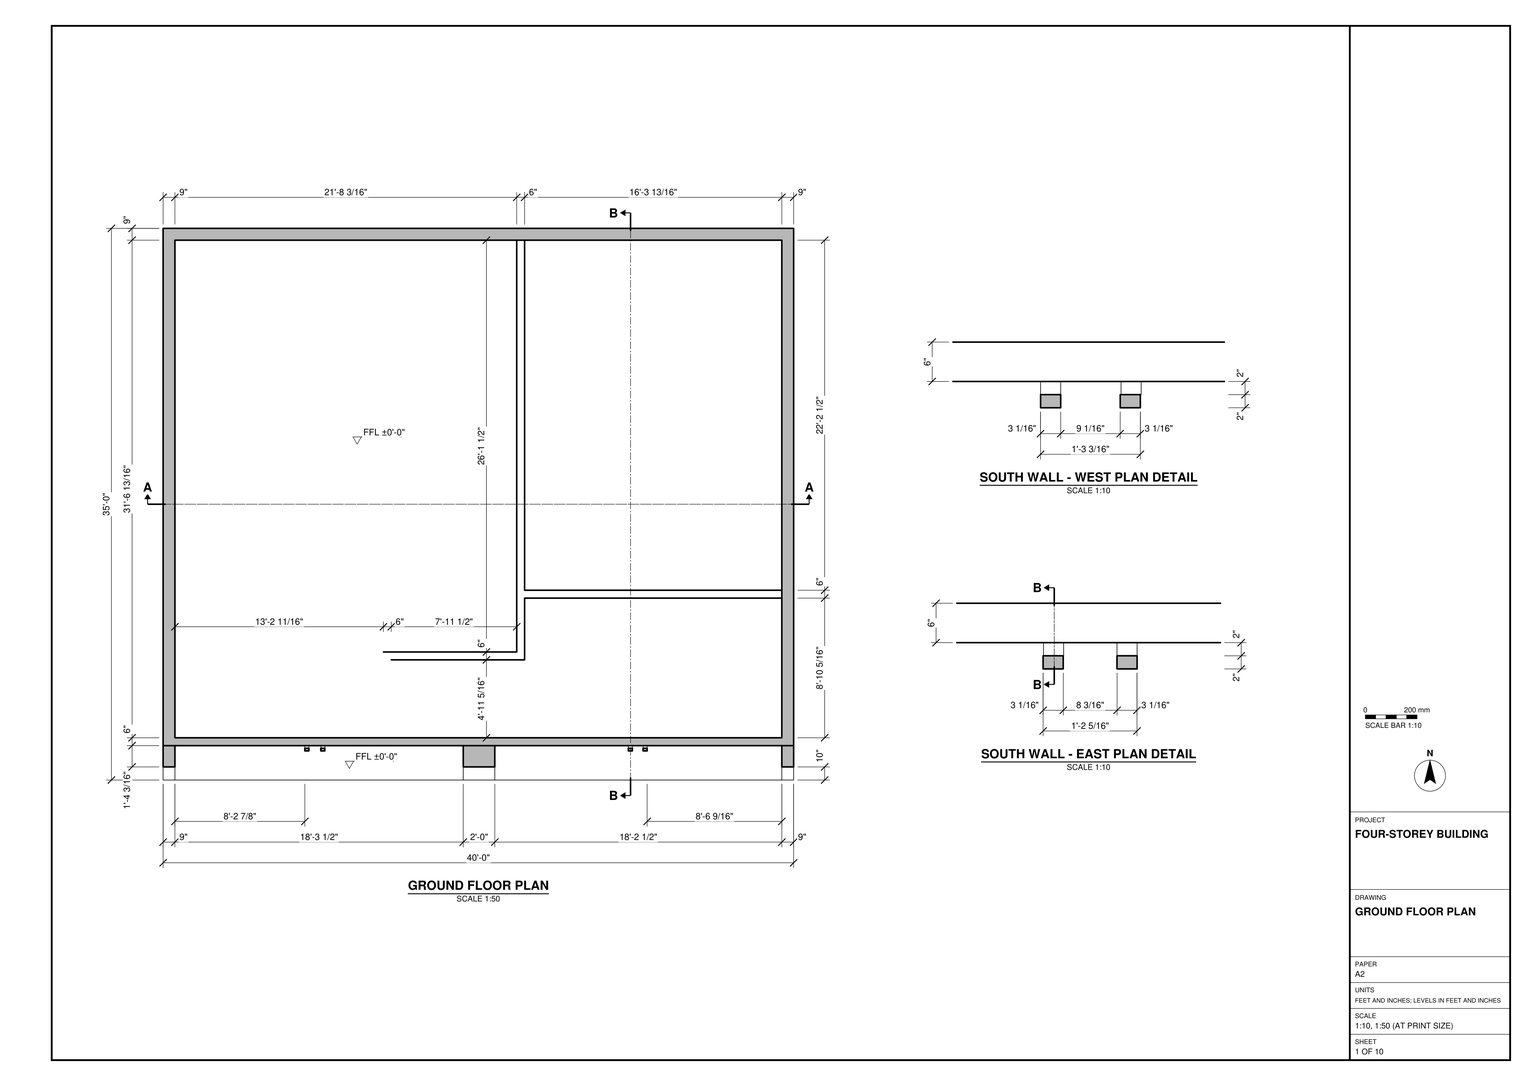
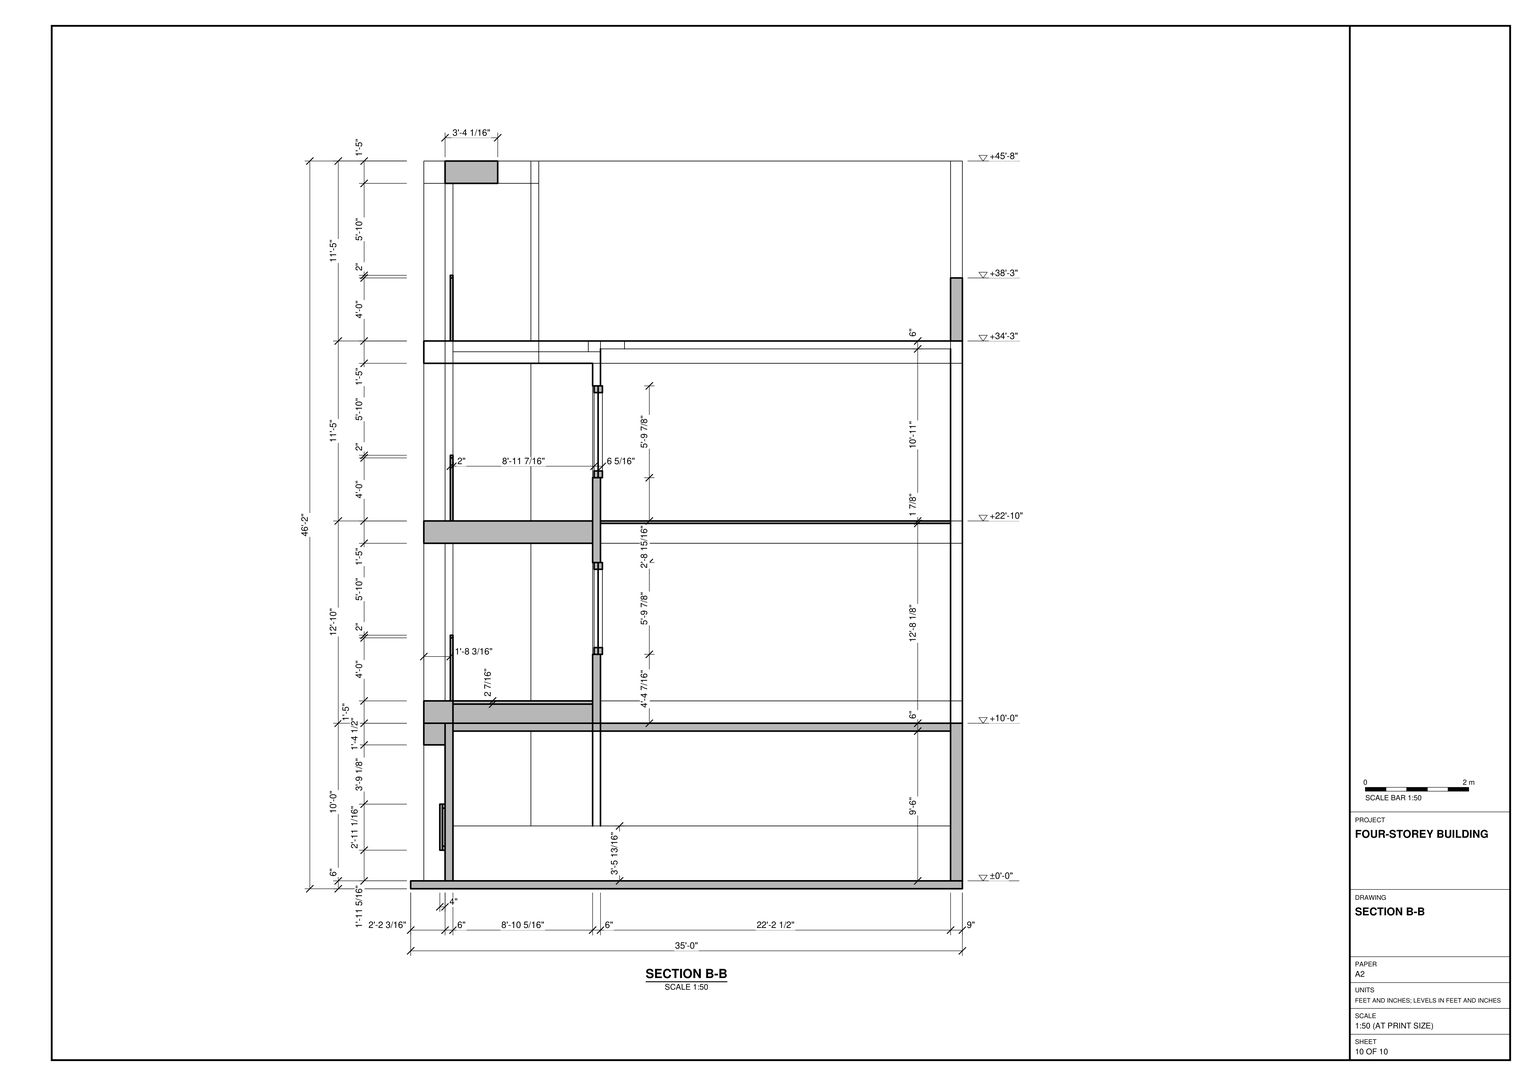
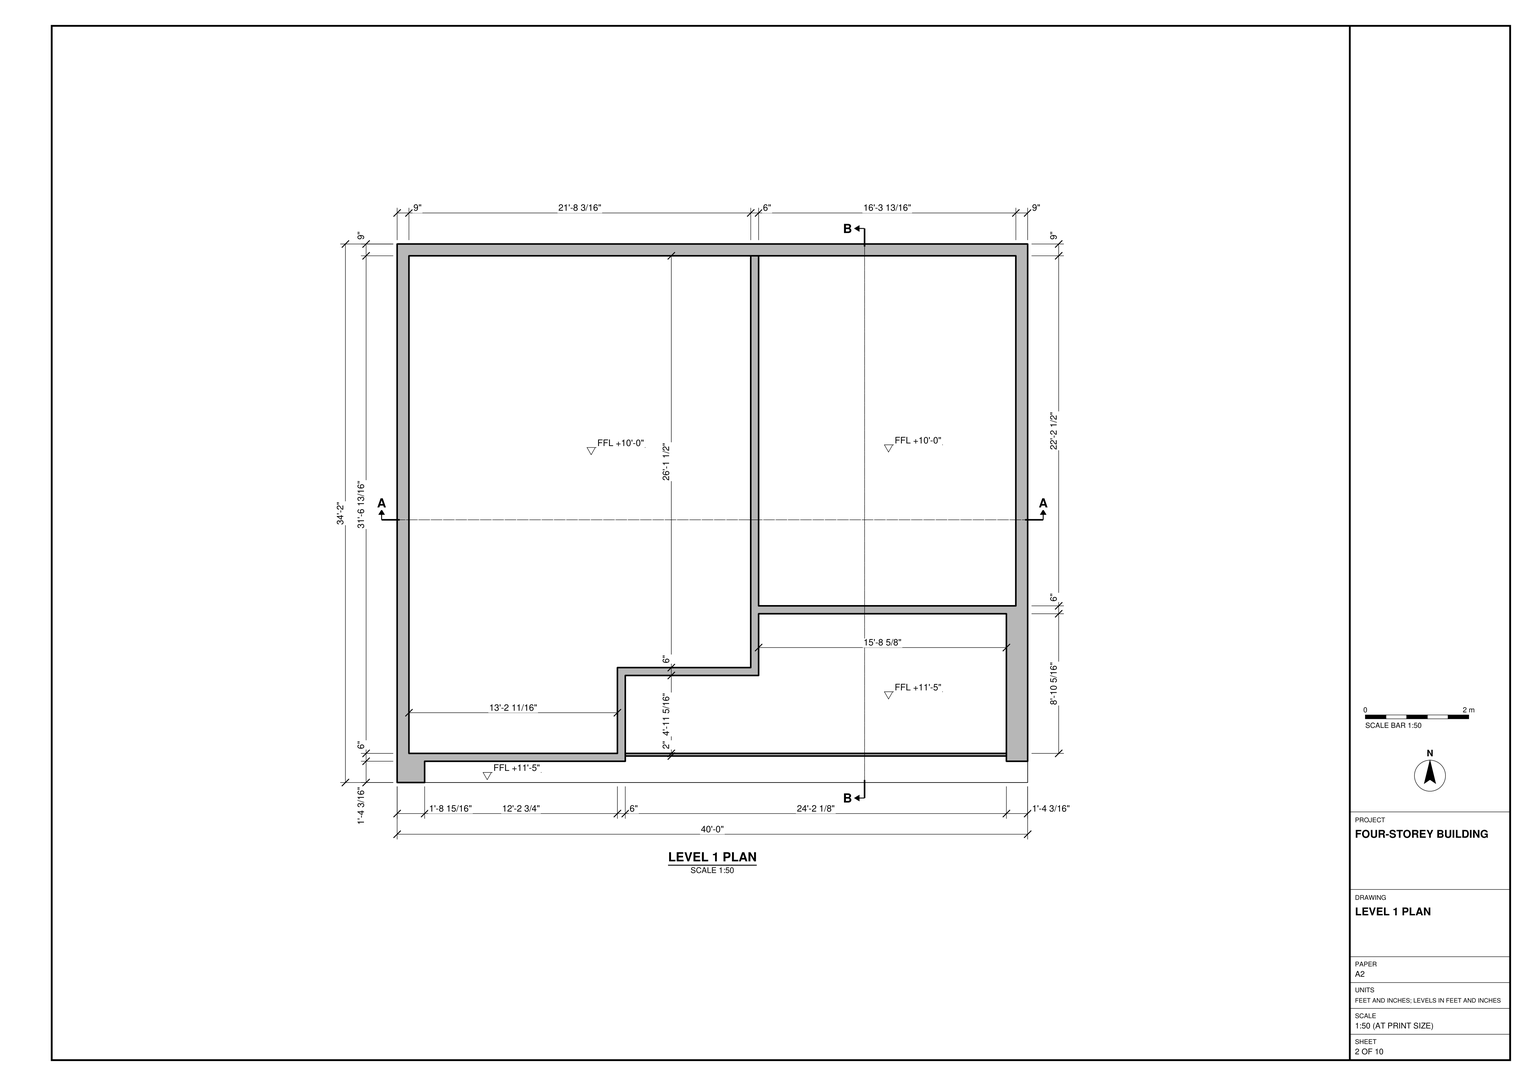
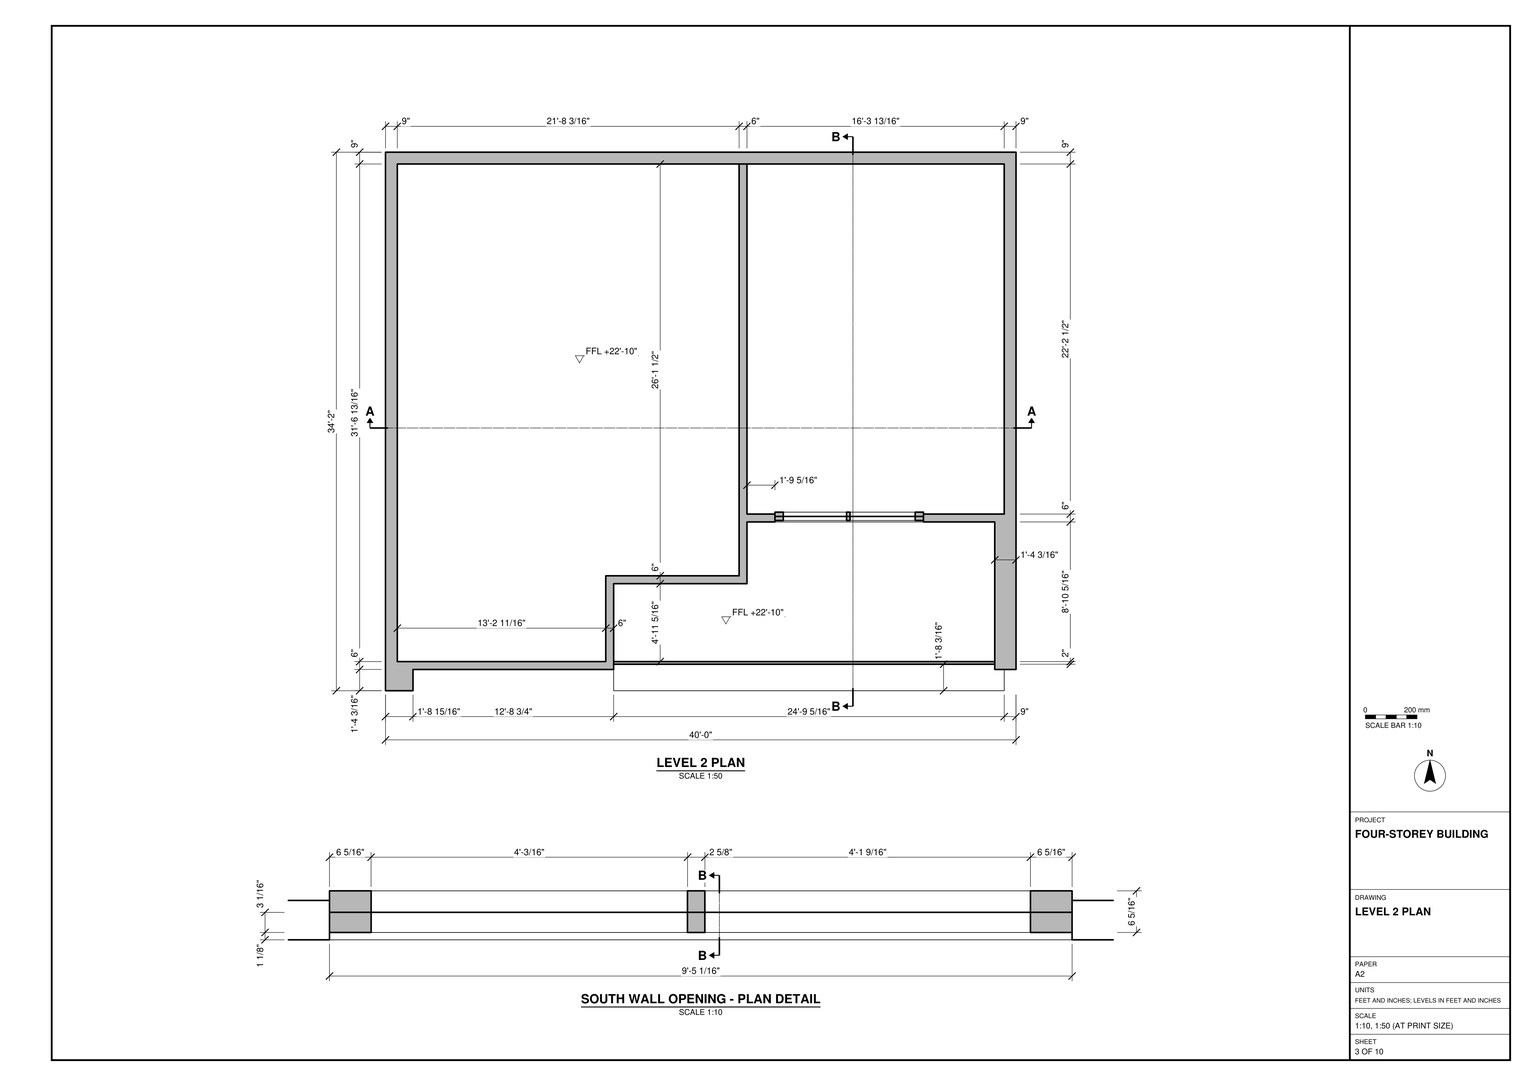
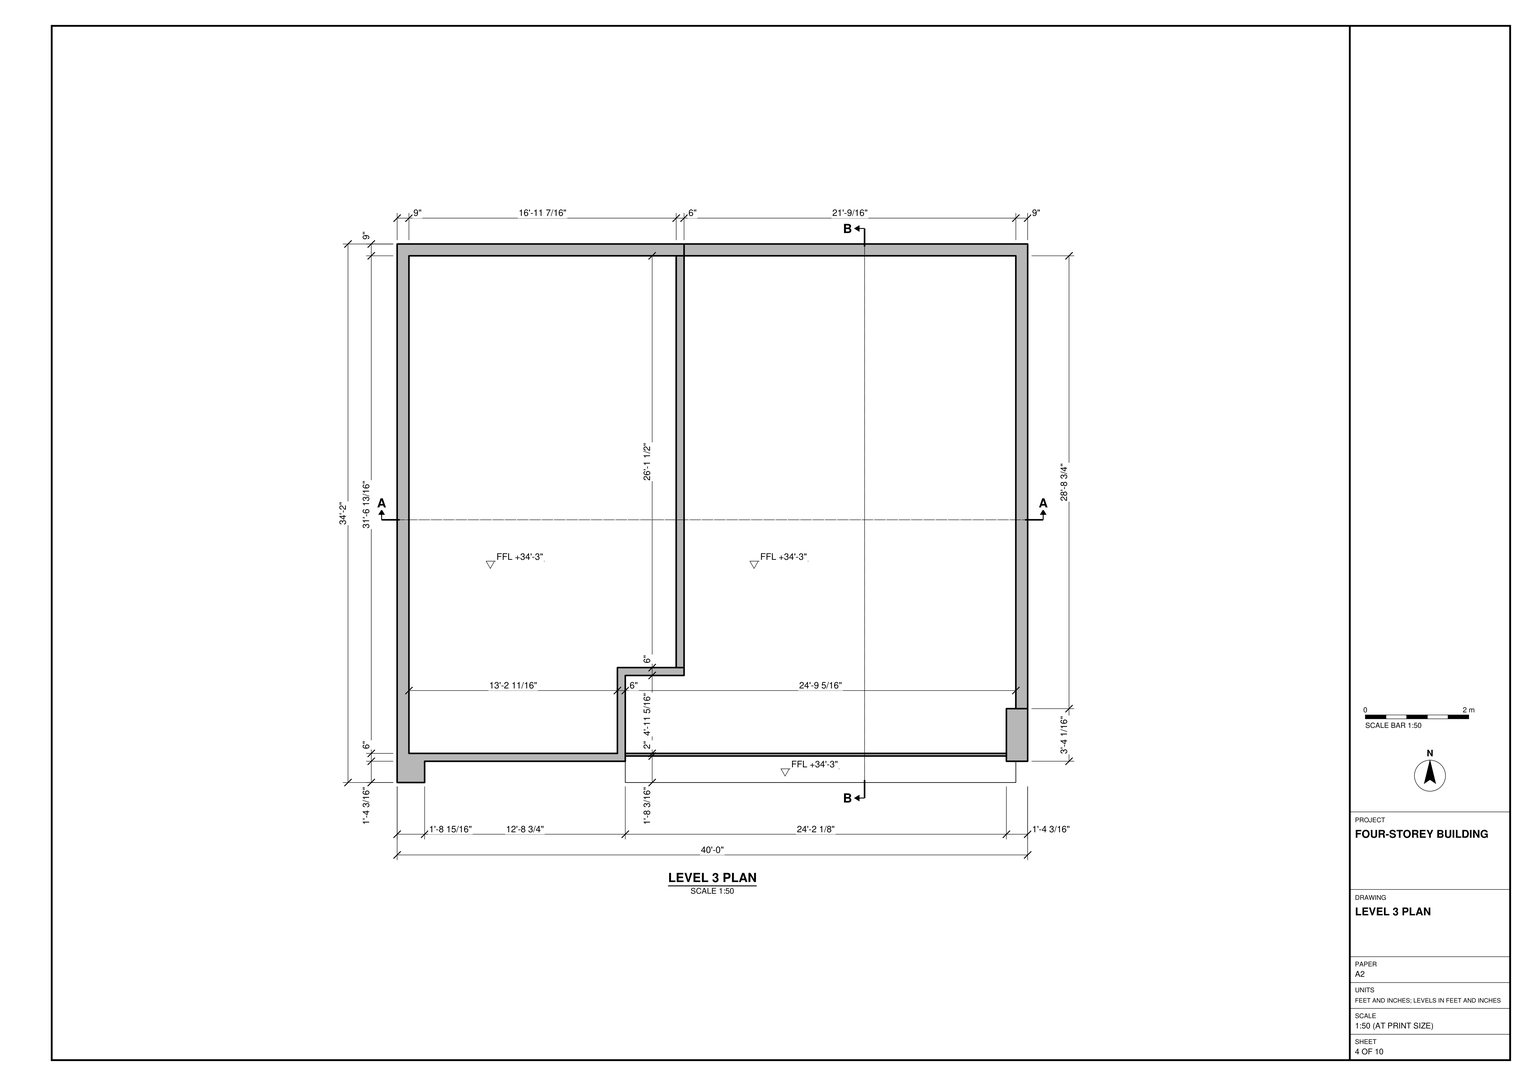
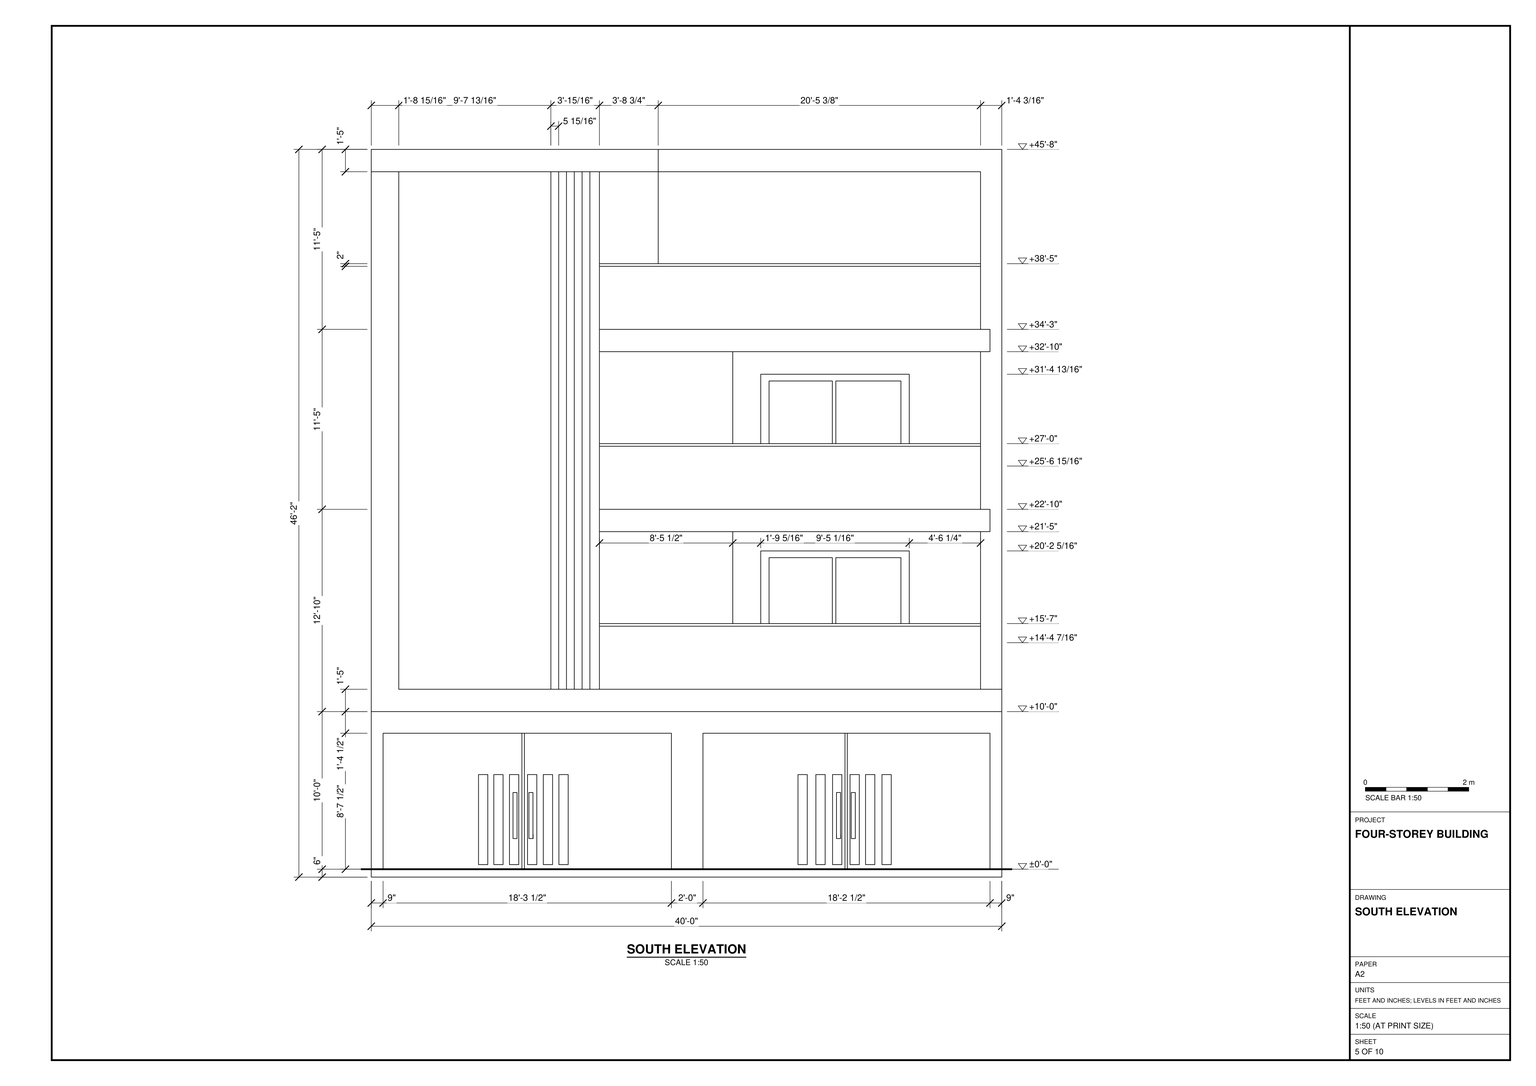
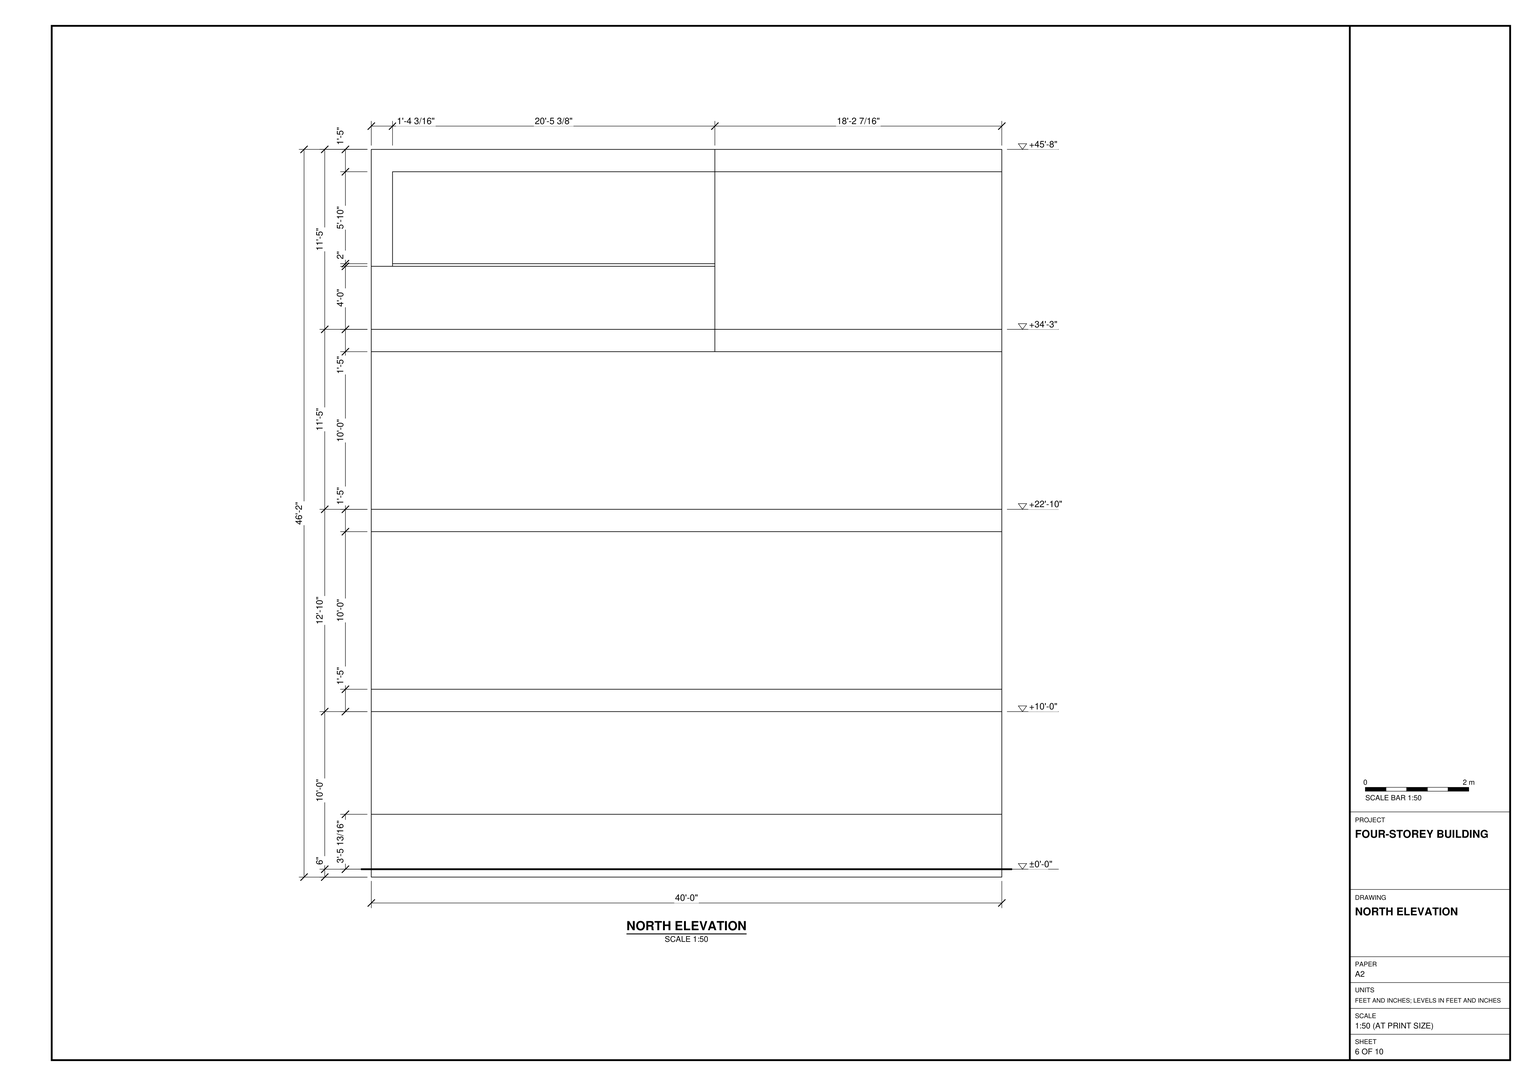
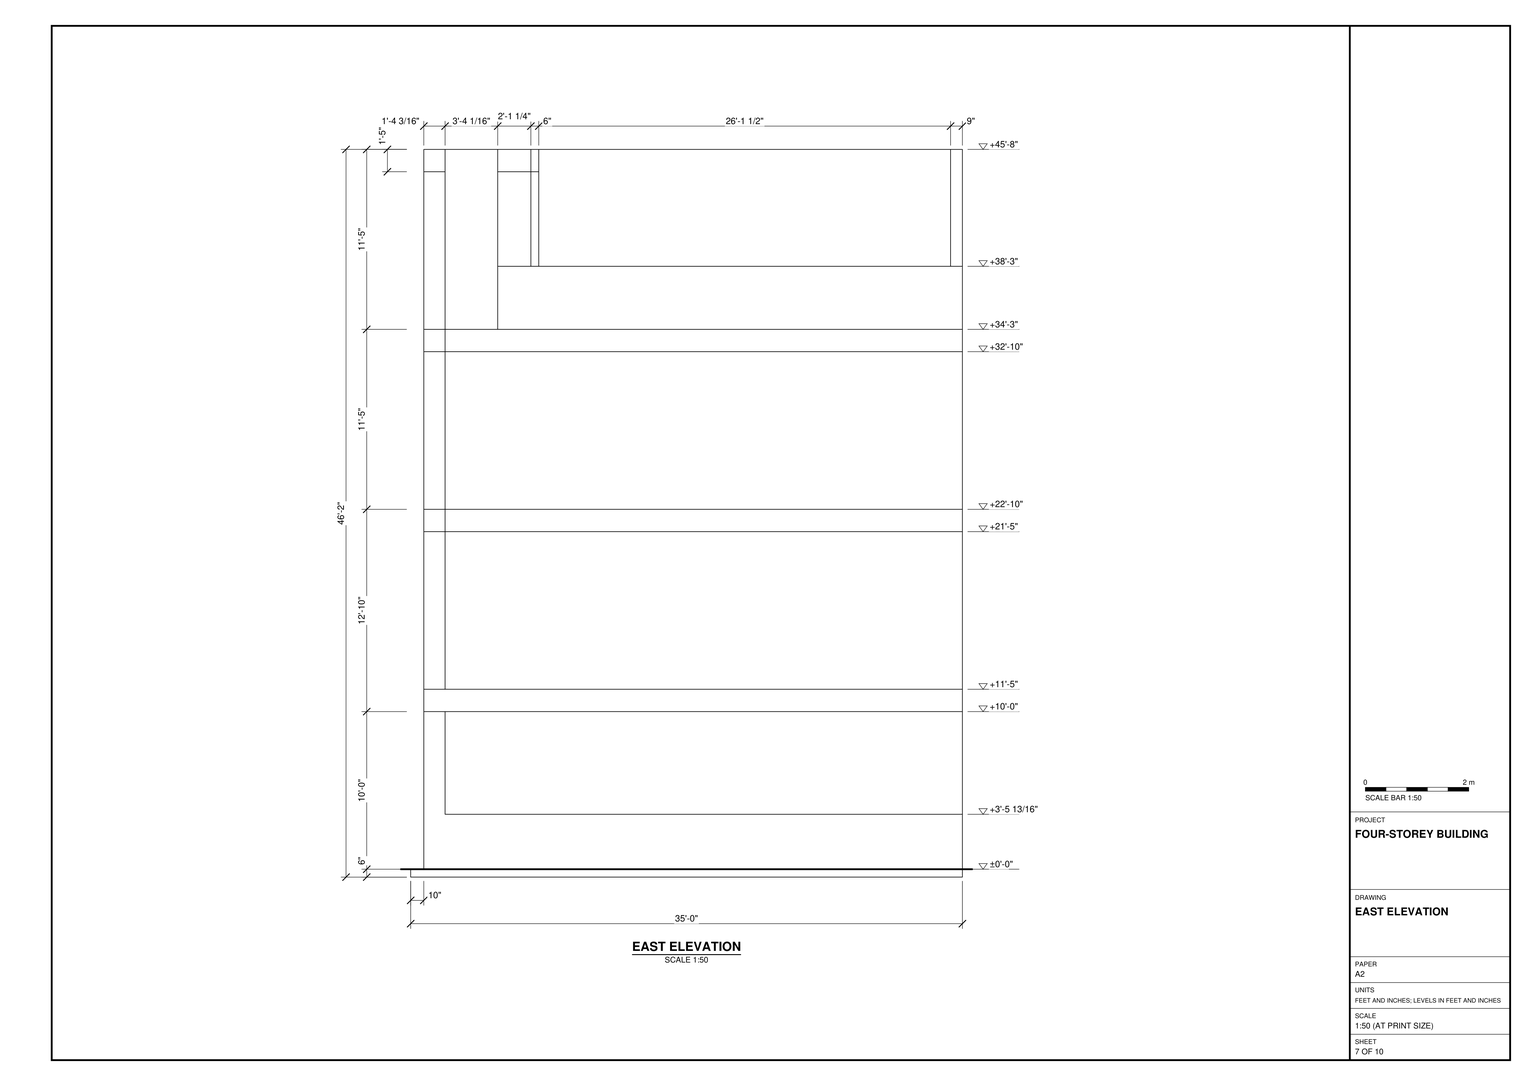
Build the four-storey building in SketchUp from task_files/diagram_01.pdf. Work in feet and inches. Set the east–west width along X to 40'-0" and the north–south depth along Y to 35'-0". The overall height is 46'-2", measured from the underside of the ground slab, not from its finished floor. Set the finished floor levels to ±0'-0", +10'-0", +22'-10" and +34'-3".

Use each floor plan for its own wall and slab outlines. Follow the wall thicknesses as drawn, including the 9" north and side walls and the 6" partitions where indicated. At the south frontage, distinguish the projecting ground slab from the stepped wall line above. Model the raised front floor area on level 1 at +11'-5" rather than continuing the +10'-0" floor through it. Use the sections to resolve slab depths, openings, guards and the roofline. Model stairs, built-in joinery and main furniture only where shown.

Keep walls, slabs and roof elements in separate groups or components. Group each furniture or joinery piece separately and use components for repeated parts. Decor and loose items, if shown, may be any suitable library components. Save one SketchUp model as output_files/four_storey_building_with_its_stepped_south_frontage.skp.

# SketchUp Ruby script. Lengths in inches.
U = 1.inch
M = Sketchup.active_model
def pt(a) = Geom::Point3d.new(a.map { |v| v * U })
def face(e, loops, mat)
  f = e.add_face(loops[0].map { |a| pt(a) })
  loops[1..].each { |l| e.add_face(l.map { |a| pt(a) }).erase! }
  f.material = f.back_material = mat if mat
  f
end
# faces: each face lists its corners as indices into pts; further lists are holes
def faces(e, pts, list, mat = nil) = list.each { |f| face(e, (f[0].is_a?(Array) ? f : [f]).map { |l| l.map { |i| pts[i] } }, mat) }
# xy, xz, yz: faces in a plane at the given z, y or x. An outline is a flat list of corners, or four numbers for a rectangle; further outlines are holes
def ring(l) = l.size == 4 ? [[l[0], l[1]], [l[2], l[1]], [l[2], l[3]], [l[0], l[3]]] : l.each_slice(2).to_a
def flat(e, list, mat, &to3) = list.each { |f| face(e, (f[0].is_a?(Array) ? f : [f]).map { |l| ring(l).map { |u, v| to3.(u, v) } }, mat) }
def xy(e, z, list, mat = nil) = flat(e, list, mat) { |x, y| [x, y, z] }
def xz(e, y, list, mat = nil) = flat(e, list, mat) { |x, z| [x, y, z] }
def yz(e, x, list, mat = nil) = flat(e, list, mat) { |y, z| [x, y, z] }
def lines(e, pts, list) = list.each { |a, b| e.add_line(pt(pts[a]), pt(pts[b])) }
# prism: a flat outline (further loops are holes) pulled along v
def prism(e, loops, v, mat = nil)
  f = face(e, loops, mat); d = Geom::Vector3d.new(v.map { |x| x * U })
  f.pushpull(f.normal.samedirection?(d) ? d.length : -d.length)
end
def box(e, o, s, mat = nil) = prism(e, [[o, [o[0] + s[0], o[1], o[2]], [o[0] + s[0], o[1] + s[1], o[2]], [o[0], o[1] + s[1], o[2]]]], [0, 0, s[2]], mat)
def at(x, y, z, deg = 0) = Geom::Transformation.translation(pt([x, y, z])) * Geom::Transformation.rotation(ORIGIN, Z_AXIS, deg.degrees)
def axes(o, x, y, z) = Geom::Transformation.new([*x, 0, *y, 0, *z, 0, *pt(o).to_a, 1])
def part(name) = M.definitions.add(name)
# library, detail: a bought-in or finely detailed component or shape, given as its bounding box
def library(name, o, s) = part(name).tap { |d| box(d.entities, o, s) }
def detail(e, o, s) = box(e.add_group.entities, o, s)
def put(e, d, t, mat = nil) = e.add_instance(d, t).tap { |i| i.material = mat if mat }
def group(e, t, mat = nil) = e.add_group.tap { |g| g.transformation = t; g.material = mat if mat }.entities
root = M.entities
M.materials.add("[Color B08]").color = [74, 25, 0]
M.materials.add("[Granite Brown]").color = [126, 104, 91]
M.materials.add("[Metal Corrugated Shiny]").color = [193, 193, 70]
M.materials.add("[Metal Silver]").color = [234, 233, 238]
M.materials.add("[Stone Brushed Khaki]").color = [226, 197, 133]
M.materials.add("[Translucent Glass Gray]").color = [128, 128, 128]
M.materials["[Translucent Glass Gray]"].alpha = 0.5
M.materials.add("[Wood Cherry Original]").color = [152, 86, 42]
M.materials.add("[Wood Floor]").color = [155, 105, 61]
M.materials.add("[Wood Veneer 01]").color = [120, 70, 37]
c1 = part("Group\#1")
xy(c1.entities,0,[[0,0,184.75,6.5625],[0,6.5625,184.75,13.5625]],"[Color B08]")
xy(c1.entities,10.36,[[10.36,0,89.06,6.5625],[93.39,0,174.39,6.5625],[10.36,6.5625,89.06,13.5625],[93.39,6.5625,174.39,13.5625]],"[Color B08]")
xy(c1.entities,131.02,[[10.36,0,89.06,6.5625],[93.39,0,174.39,6.5625],[10.36,6.5625,89.06,13.5625],[93.39,6.5625,174.39,13.5625]],"[Color B08]")
xy(c1.entities,141.375,[[0,0,184.75,6.5625],[0,6.5625,184.75,13.5625]],"[Color B08]")
xz(c1.entities,0,[[[0,0,184.75,141.375],[93.39,10.36,174.39,131.02],[10.36,10.36,89.06,131.02]]],"[Color B08]")
xz(c1.entities,6.5625,[[[0,0,184.75,141.375],[93.39,10.36,174.39,131.02],[10.36,10.36,89.06,131.02]]],"[Color B08]")
xz(c1.entities,6.5625,[[10.36,10.36,89.06,131.02],[93.39,10.36,174.39,131.02]],"[Translucent Glass Gray]")
xz(c1.entities,13.5625,[[[0,0,184.75,141.375],[93.39,10.36,174.39,131.02],[10.36,10.36,89.06,131.02]]],"[Color B08]")
yz(c1.entities,0,[[0,0,6.5625,141.375],[6.5625,0,13.5625,141.375]],"[Color B08]")
yz(c1.entities,10.36,[[0,10.36,6.5625,131.02],[6.5625,10.36,13.5625,131.02]],"[Color B08]")
yz(c1.entities,89.06,[[0,10.36,6.5625,131.02],[6.5625,10.36,13.5625,131.02]],"[Color B08]")
yz(c1.entities,93.39,[[0,10.36,6.5625,131.02],[6.5625,10.36,13.5625,131.02]],"[Color B08]")
yz(c1.entities,174.39,[[0,10.36,6.5625,131.02],[6.5625,10.36,13.5625,131.02]],"[Color B08]")
yz(c1.entities,184.75,[[0,0,6.5625,141.375],[6.5625,0,13.5625,141.375]],"[Color B08]")
xy(root,0,[[0,0,480,420]])
xy(root,6,[[[0,10,0,420,480,420,480,10,471,10,471,26.1875,9,26.1875,9,10],[9,32.1875,471,411]],[228.48,10,252.5,26.1875],[9,32.1875,471,411]])
xy(root,6,[[0,0,9,10],[9,0,228.48,26.1875],[228.48,0,252.5,10],[252.5,0,471,26.1875],[471,0,480,10]],"[Stone Brushed Khaki]")
xy(root,29.34,[[354.15,22.1875,357.21,24.1875],[365.4,22.1875,368.46,24.1875],[354.21,24.1875,357.28,26.1875],[365.4,24.1875,368.46,26.1875]])
xy(root,29.34,[[107.9,22.1875,110.96,24.1875],[120.03,22.1875,123.09,24.1875],[107.9,24.1875,110.96,26.1875],[120.15,24.1875,123.21,26.1875]],"[Metal Corrugated Shiny]")
xy(root,32.41,[[107.9,24.1875,110.96,26.1875],[120.15,24.1875,123.21,26.1875],[354.21,24.1875,357.28,26.1875],[365.4,24.1875,368.46,26.1875]],"[Metal Corrugated Shiny]")
xy(root,61.34,[[107.9,24.1875,110.96,26.1875],[354.15,24.1875,357.21,26.1875],[365.4,24.1875,368.46,26.1875]])
xy(root,61.34,[[120.03,24.1875,123.09,26.1875]],"[Wood Floor]")
xy(root,64.41,[[107.9,22.1875,110.96,26.1875],[120.03,22.1875,123.09,26.1875],[354.15,22.1875,357.21,24.1875],[365.4,22.1875,368.46,24.1875],[354.15,24.1875,357.21,26.1875],
  [365.4,24.1875,368.46,26.1875]],"[Metal Corrugated Shiny]")
xy(root,109.52,[[9,10,228.48,26.1875],[252.5,10,471,26.1875]],"[Stone Brushed Khaki]")
xy(root,120,[[9,32.1875,471,411]])
xy(root,126,[[0,10,9,26.1875],[9,10,173.6875,26.1875],[173.6875,10,471,26.1875],[471,10,480,26.1875],[[0,26.1875,0,420,480,420,480,26.1875,173.6875,26.1875,173.6875,32.1875,471,32.1875,471,138.5,275.1875,138.5,275.1875,91.5,173.6875,91.5,173.6875,26.1875],[9,32.1875,167.6875,32.1875,167.6875,97.5,269.1875,97.5,269.1875,411,9,411],[275.1875,144.5,471,411]],
  [9,32.1875,167.6875,32.1875,167.6875,97.5,269.1875,97.5,269.1875,411,9,411],[173.6875,32.1875,471,32.1875,471,138.5,275.1875,138.5,275.1875,91.5,173.6875,91.5],[275.1875,144.5,471,411]])
xy(root,140.5625,[[173.6875,32.1875,173.6875,91.5,275.1875,91.5,275.1875,138.5,471,138.5,471,32.1875]])
xy(root,143,[[173.6875,30.1875,463.8125,32.1875],[173.6875,32.1875,463.8125,32.1875,463.8125,138.5,275.1875,138.5,275.1875,91.5,173.6875,91.5],[463.8125,32.1875,471,138.5]])
xy(root,143,[[20.9375,10,480,10,480,26.1875,463.8125,26.1875,463.8125,30.1875,173.6875,30.1875,173.6875,26.1875,20.9375,26.1875]],"[Wood Cherry Original]")
xy(root,178.45,[[296.49,138.5,409.55,144.5]])
xy(root,191,[[173.6875,30.1875,463.8125,32.1875]])
xy(root,193,[[173.6875,30.1875,463.8125,32.1875]],"[Metal Silver]")
xy(root,248.32,[[296.49,138.5,409.55,144.5]])
xy(root,263,[[173.6875,10,275.1875,91.5],[275.1875,10,275.1875,138.5,463.8125,138.5,463.8125,26.1875,471,26.1875,471,10],[463.8125,26.1875,471,32.1875],[463.8125,32.1875,471,138.5]])
xy(root,274,[[9,32.1875,9,411,269.1875,411,269.1875,97.5,167.6875,97.5,167.6875,32.1875]])
xy(root,278.125,[[275.1875,144.5,471,411]])
xy(root,280,[[463.8125,26.1875,471,32.1875],[173.6875,30.1875,463.8125,32.1875],[9,32.1875,167.6875,32.1875,167.6875,97.5,269.1875,97.5,269.1875,411,9,411],[173.6875,32.1875,463.8125,32.1875,463.8125,138.5,275.1875,138.5,275.1875,91.5,173.6875,91.5],[463.8125,32.1875,471,138.5],
  [275.1875,144.5,471,411]])
xy(root,280,[[173.6875,10,471,10,471,26.1875,463.8125,26.1875,463.8125,30.1875,173.6875,30.1875]],"[Wood Cherry Original]")
xy(root,312.95,[[296.49,138.5,409.55,144.5]])
xy(root,328,[[173.6875,30.1875,463.8125,32.1875]])
xy(root,330,[[173.6875,30.1875,463.8125,32.1875]],"[Metal Silver]")
xy(root,382.82,[[296.49,138.5,409.55,144.5]])
xy(root,400,[[173.6875,10,173.6875,91.5,275.1875,91.5,275.1875,138.5,463.8125,138.5,463.8125,26.1875,471,26.1875,471,10]])
xy(root,408.8125,[[9,32.1875,9,411,269.1875,411,269.1875,97.5,167.6875,97.5,167.6875,32.1875]])
xy(root,417,[[173.6875,10,471,10,471,26.1875,463.8125,26.1875,463.8125,30.1875,173.6875,30.1875],[173.6875,30.1875,463.8125,32.1875],[9,32.1875,167.6875,32.1875,167.6875,97.5,212.4375,97.5,212.4375,411,9,411],[173.6875,32.1875,463.8125,32.1875,463.8125,66.25,471,66.25,471,411,218.4375,411,218.4375,91.5,173.6875,91.5],[471,66.25,471,411,218.4375,411,218.4375,420,480,420,480,66.25],
  [212.4375,97.5,218.4375,411]])
xy(root,465,[[173.6875,30.1875,463.8125,32.1875],[471,66.25,480,66.25,480,420,218.4375,420,218.4375,411,471,411]])
xy(root,467,[[173.6875,30.1875,463.8125,32.1875]],"[Metal Silver]")
xy(root,537,[[218.4375,26.1875,463.8125,66.25]])
xy(root,537,[[20.9375,10,20.9375,26.1875,173.6875,26.1875,173.6875,91.5,218.4375,91.5,218.4375,10]],"[Wood Cherry Original]")
xy(root,548,[[9,32.1875,9,411,212.4375,411,212.4375,97.5,167.6875,97.5,167.6875,32.1875]])
xy(root,554,[[0,10,218.4375,420],[218.4375,26.1875,480,66.25]])
xz(root,0,[[0,0,480,6]],"[Stone Brushed Khaki]")
xz(root,10,[[173.6875,400,471,417]])
xz(root,10,[[0,6,9,6,9,109.52,228.48,109.52,228.48,6,252.5,6,252.5,109.52,471,109.52,471,6,480,6,480,126,0,126]],"[Stone Brushed Khaki]")
xz(root,10,[[0,126,480,126,480,143,20.9375,143,20.9375,537,0,537],[173.6875,263,471,280],[0,537,218.4375,554]],"[Wood Cherry Original]")
xz(root,22.1875,[[107.9,29.34,110.96,64.41],[120.03,29.34,123.09,64.41],[354.15,29.34,357.21,64.41],[365.4,29.34,368.46,64.41]],"[Metal Corrugated Shiny]")
xz(root,24.1875,[[107.9,29.34,110.96,30.875],[354.21,29.34,357.21,30.875],[357.21,29.34,357.28,30.875],[365.4,29.34,368.46,30.875],[107.9,30.875,110.96,32.41],
  [354.21,30.875,357.21,32.41],[357.21,30.875,357.28,32.41],[365.4,30.875,368.46,32.41],[354.15,61.34,357.21,64.41],[365.4,61.34,368.46,64.41]])
xz(root,24.1875,[[120.03,29.34,120.03,61.34,123.09,61.34,123.09,32.41,120.15,32.41,120.15,29.34],[354.15,29.34,354.15,61.34,357.21,61.34,357.21,32.41,354.21,32.41,354.21,29.34],[107.9,32.41,110.96,61.34],[365.4,32.41,368.46,61.34]],"[Metal Corrugated Shiny]")
xz(root,24.1875,[[120.15,29.34,123.09,30.875],[123.09,29.34,123.21,30.875],[120.15,30.875,123.09,32.41],[123.09,30.875,123.21,32.41]],"[Wood Floor]")
xz(root,26.1875,[[228.48,6,228.48,109.52,9,109.52,9,126,471,126,471,109.52,252.5,109.52,252.5,6],[114.68,6,116.55,109.52],[107.9,29.34,110.96,32.41],[354.21,29.34,357.28,32.41],[365.4,29.34,368.46,32.41],
  [0,47.8125,9,126],[471,47.8125,480,126],[107.9,61.34,110.96,64.41],[354.15,61.34,357.21,64.41],[365.4,61.34,368.46,64.41],
  [463.8125,143,480,143,480,554,218.4375,554,218.4375,537,463.8125,537,463.8125,417,471,417,471,400,463.8125,400,463.8125,280,471,280,471,263,463.8125,263]])
xz(root,26.1875,[[20.9375,143,136.73,537],[136.73,143,142.67,537],[142.67,143,148.6,537],[148.6,143,154.54,537],[154.54,143,160.48,537],
  [160.48,143,166.42,537],[166.42,143,173.6875,537]],"[Granite Brown]")
xz(root,26.1875,[[360.625,6,362.375,109.52],[81.65,9.5,88.71,78.06],[93.28,9.5,100.34,78.06],[[105.21,9.5,112.28,78.06],[107.9,61.34,110.96,64.41],[107.9,29.34,110.96,32.41]],[[118.96,9.5,126.03,78.06],[120.03,61.34,123.09,64.41],[120.15,29.34,123.21,32.41]],
  [130.96,9.5,138.03,78.06],[142.84,9.5,149.9,78.06],[324.84,9.5,331.9,78.06],[338.46,9.5,345.53,78.06],[[351.15,9.5,358.21,78.06],[354.15,61.34,357.21,64.41],[354.21,29.34,357.28,32.41]],
  [[364.46,9.5,371.53,78.06],[365.4,61.34,368.46,64.41],[365.4,29.34,368.46,32.41]],[376.28,9.5,383.34,78.06],[388.78,9.5,395.84,78.06],[120.15,29.34,123.21,32.41],[120.03,61.34,123.09,64.41]],"[Wood Floor]")
xz(root,26.1875,[[[9,6,114.68,109.52],[105.21,9.5,112.28,78.06],[93.28,9.5,100.34,78.06],[81.65,9.5,88.71,78.06]],[[116.55,6,228.48,109.52],[118.96,9.5,126.03,78.06],[130.96,9.5,138.03,78.06],[142.84,9.5,149.9,78.06]],[[252.5,6,360.625,109.52],[351.15,9.5,358.21,78.06],[338.46,9.5,345.53,78.06],[324.84,9.5,331.9,78.06]],[[362.375,6,471,109.52],[364.46,9.5,371.53,78.06],[376.28,9.5,383.34,78.06],[388.78,9.5,395.84,78.06]]],"[Wood Veneer 01]")
xz(root,30.1875,[[173.6875,191,463.8125,193],[173.6875,328,463.8125,330],[173.6875,465,463.8125,467]],"[Metal Silver]")
xz(root,30.1875,[[173.6875,143,463.8125,191],[173.6875,280,463.8125,328],[173.6875,417,463.8125,465]],"[Translucent Glass Gray]")
xz(root,32.1875,[[9,6,9,47.8125,167.6875,47.8125,167.6875,120,173.6875,120,173.6875,47.8125,471,47.8125,471,6],[9,47.8125,167.6875,120],[173.6875,47.8125,471,120],[9,120,167.6875,126],[173.6875,120,471,126],
  [9,126,167.6875,143],[173.6875,126,471,140.5625],[173.6875,140.5625,471,143],[9,143,167.6875,263],[9,263,167.6875,274],
  [9,274,167.6875,280],[9,280,167.6875,400],[9,400,167.6875,408.8125],[9,408.8125,167.6875,417],[9,417,167.6875,537],
  [9,537,167.6875,548]])
xz(root,32.1875,[[173.6875,191,463.8125,193],[173.6875,328,463.8125,330],[173.6875,465,463.8125,467]],"[Metal Silver]")
xz(root,32.1875,[[173.6875,143,463.8125,191],[173.6875,280,463.8125,328],[173.6875,417,463.8125,465]],"[Translucent Glass Gray]")
xz(root,66.25,[[463.8125,417,463.8125,537,218.4375,537,218.4375,554,480,554,480,465,471,465,471,417],[471,417,480,465]])
xz(root,91.5,[[173.6875,47.8125,275.1875,126],[173.6875,126,275.1875,140.5625],[173.6875,140.5625,194.1875,143],[194.1875,140.5625,275.1875,143],[173.6875,263,275.1875,280]])
xz(root,91.5,[[173.6875,143,275.1875,263],[173.6875,280,275.1875,400],[173.6875,417,218.4375,537]],"[Granite Brown]")
xz(root,97.5,[[167.6875,47.8125,269.1875,126],[167.6875,126,269.1875,143],[167.6875,143,269.1875,263],[167.6875,263,269.1875,274],[167.6875,274,269.1875,280],
  [167.6875,280,269.1875,400],[167.6875,400,218.4375,408.8125],[218.4375,400,269.1875,408.8125],[167.6875,408.8125,218.4375,417],[167.6875,417,212.4375,537],
  [212.4375,417,218.4375,537],[167.6875,537,212.4375,548]])
xz(root,138.5,[[275.1875,47.8125,471,126],[275.1875,126,471,140.5625],[275.1875,140.5625,471,143],[275.1875,263,471,280]])
xz(root,138.5,[[[275.1875,143,463.8125,263],[296.49,178.45,409.55,248.32]],[[275.1875,280,463.8125,400],[296.49,312.95,409.55,382.82]]],"[Granite Brown]")
xz(root,144.5,[[275.1875,47.8125,471,126],[275.1875,126,471,143],[[275.1875,143,471,263],[296.49,178.45,409.55,248.32]],[275.1875,263,471,278.125],[275.1875,278.125,471,280],
  [[275.1875,280,471,400],[296.49,312.95,409.55,382.82]],[275.1875,400,471,411]])
xz(root,411,[[9,6,471,6,471,47.8125,275.1875,47.8125,275.1875,120,269.1875,120,269.1875,47.8125,9,47.8125],[9,47.8125,25.0625,120],[25.0625,47.8125,269.1875,120],[275.1875,47.8125,471,120],[9,120,25.0625,126],
  [25.0625,120,269.1875,126],[269.1875,120,275.1875,417],[275.1875,120,471,126],[9,126,269.1875,143],[275.1875,126,471,143],
  [9,143,269.1875,263],[275.1875,143,471,263],[9,263,269.1875,274],[275.1875,263,471,278.125],[9,274,18.84,280],
  [18.84,274,27.21,280],[27.21,274,269.1875,280],[275.1875,278.125,310.71,280],[310.71,278.125,320.71,280],[320.71,278.125,471,280],
  [9,280,269.1875,400],[275.1875,280,471,400],[9,400,218.4375,408.8125],[218.4375,400,269.1875,408.8125],[275.1875,400,471,411],
  [9,408.8125,218.4375,417],[218.4375,408.8125,269.1875,417],[9,417,212.4375,537],[212.4375,417,218.4375,537],[218.4375,417,471,465],
  [9,537,212.4375,548]])
xz(root,420,[[0,0,480,6],[0,6,480,47.8125],[0,47.8125,480,126],[0,126,480,143],[0,143,480,263],
  [0,263,480,280],[0,280,480,400],[0,400,218.4375,417],[218.4375,400,480,417],[0,417,218.4375,537],
  [218.4375,417,480,465],[0,537,218.4375,554]])
yz(root,0,[[0,0,420,6],[10,6,10,126,26.1875,126,26.1875,47.8125,420,47.8125,420,6],[26.1875,47.8125,420,126],[10,126,420,143],[10,143,420,263],
  [10,263,420,280],[10,280,420,400],[10,400,420,417],[10,417,420,537],[10,537,420,554]])
yz(root,9,[[32.1875,6,411,47.8125],[32.1875,47.8125,411,120],[32.1875,120,411,126],[32.1875,126,411,143],[32.1875,143,411,263],
  [32.1875,263,411,274],[32.1875,274,411,280],[32.1875,280,411,400],[32.1875,400,411,408.8125],[32.1875,408.8125,135.22,417],
  [135.22,408.8125,162.78,417],[162.78,408.8125,411,417],[32.1875,417,411,537],[32.1875,537,411,548]])
yz(root,9,[[10,6,26.1875,109.52]],"[Stone Brushed Khaki]")
yz(root,20.9375,[[10,143,26.1875,537]],"[Wood Cherry Original]")
yz(root,107.9,[[24.1875,29.34,26.1875,32.41]])
yz(root,107.9,[[22.1875,29.34,22.1875,64.41,26.1875,64.41,26.1875,61.34,24.1875,61.34,24.1875,29.34]],"[Metal Corrugated Shiny]")
yz(root,110.96,[[22.1875,29.34,24.1875,62.875],[24.1875,29.34,26.1875,32.41],[24.1875,61.34,26.1875,64.41],[22.1875,62.875,24.1875,64.41]],"[Metal Corrugated Shiny]")
yz(root,120.03,[[22.1875,29.34,22.1875,64.41,26.1875,64.41,26.1875,61.34,24.1875,61.34,24.1875,29.34]],"[Metal Corrugated Shiny]")
yz(root,120.15,[[24.1875,29.34,26.1875,32.41]],"[Metal Corrugated Shiny]")
yz(root,123.09,[[22.1875,29.34,24.1875,29.34,24.1875,61.34,26.1875,61.34,26.1875,64.41,22.1875,64.41]],"[Metal Corrugated Shiny]")
yz(root,123.21,[[24.1875,29.34,26.1875,32.41]],"[Metal Corrugated Shiny]")
yz(root,167.6875,[[32.1875,126,97.5,143],[32.1875,143,97.5,263],[32.1875,263,97.5,274],[32.1875,274,97.5,280],[32.1875,280,97.5,400],
  [32.1875,400,97.5,408.8125],[32.1875,408.8125,97.5,417],[32.1875,417,97.5,537],[32.1875,537,97.5,548]])
yz(root,173.6875,[[32.1875,126,91.5,140.5625],[32.1875,140.5625,91.5,143],[30.1875,143,32.1875,191],[30.1875,191,32.1875,193],[26.1875,263,32.1875,280],
  [32.1875,263,91.5,280],[30.1875,280,32.1875,328],[30.1875,328,32.1875,330],[10,400,26.1875,417],[30.1875,417,32.1875,465],
  [30.1875,465,32.1875,467]])
yz(root,173.6875,[[26.1875,143,30.1875,143,30.1875,193,32.1875,193,32.1875,263,26.1875,263],[32.1875,143,91.5,263],[26.1875,280,30.1875,280,30.1875,330,32.1875,330,32.1875,400,26.1875,400],[32.1875,280,91.5,400],[26.1875,417,30.1875,417,30.1875,467,32.1875,467,32.1875,537,26.1875,537],
  [32.1875,417,91.5,537]],"[Granite Brown]")
yz(root,173.6875,[[10,263,26.1875,280]],"[Wood Cherry Original]")
yz(root,212.4375,[[97.5,417,411,548]])
yz(root,218.4375,[[411,400,420,417],[91.5,417,97.5,537],[411,417,420,465],[411,465,420,554],[26.1875,537,66.25,554],
  [91.5,537,97.5,554]])
yz(root,218.4375,[[97.5,417,411,554]],"[Granite Brown]")
yz(root,218.4375,[[10,537,26.1875,554],[66.25,537,91.5,554]],"[Wood Cherry Original]")
yz(root,228.48,[[10,6,26.1875,109.52]],"[Stone Brushed Khaki]")
yz(root,252.5,[[10,6,26.1875,109.52]],"[Stone Brushed Khaki]")
yz(root,269.1875,[[97.5,47.8125,411,126],[97.5,126,411,143],[97.5,143,411,263],[97.5,263,411,274],[97.5,274,411,280],
  [97.5,280,411,400],[97.5,400,411,408.8125]])
yz(root,275.1875,[[91.5,47.8125,138.5,126],[144.5,47.8125,411,126],[91.5,126,138.5,140.5625],[144.5,126,411,143],[91.5,140.5625,138.5,143],
  [144.5,143,411,263],[91.5,263,138.5,280],[144.5,263,411,278.125],[144.5,278.125,411,280],[144.5,280,411,400],
  [144.5,400,411,411]])
yz(root,275.1875,[[91.5,143,138.5,263],[91.5,280,138.5,400]],"[Granite Brown]")
yz(root,296.49,[[138.5,178.45,144.5,248.32],[138.5,312.95,144.5,382.82]])
yz(root,354.15,[[22.1875,29.34,24.1875,64.41],[24.1875,61.34,26.1875,64.41]],"[Metal Corrugated Shiny]")
yz(root,354.21,[[24.1875,29.34,26.1875,32.41]],"[Metal Corrugated Shiny]")
yz(root,357.21,[[22.1875,29.34,24.1875,64.41],[24.1875,61.34,26.1875,64.41]],"[Metal Corrugated Shiny]")
yz(root,357.28,[[24.1875,29.34,26.1875,32.41]],"[Metal Corrugated Shiny]")
yz(root,365.4,[[22.1875,29.34,24.1875,64.41],[24.1875,29.34,26.1875,32.41],[24.1875,61.34,26.1875,64.41]],"[Metal Corrugated Shiny]")
yz(root,368.46,[[22.1875,29.34,24.1875,64.41],[24.1875,29.34,26.1875,32.41],[24.1875,61.34,26.1875,64.41]],"[Metal Corrugated Shiny]")
yz(root,409.55,[[138.5,178.45,144.5,248.32],[138.5,312.95,144.5,382.82]])
yz(root,463.8125,[[30.1875,143,32.1875,191],[30.1875,191,32.1875,193],[30.1875,280,32.1875,328],[30.1875,328,32.1875,330],[26.1875,417,26.1875,537,66.25,537,66.25,417,32.1875,417,32.1875,467,30.1875,467,30.1875,417],
  [30.1875,417,32.1875,465],[30.1875,465,32.1875,467]])
yz(root,463.8125,[[26.1875,143,26.1875,263,138.5,263,138.5,143,32.1875,143,32.1875,193,30.1875,193,30.1875,143],[26.1875,280,26.1875,400,138.5,400,138.5,280,32.1875,280,32.1875,330,30.1875,330,30.1875,280]],"[Granite Brown]")
yz(root,471,[[32.1875,6,32.1875,47.8125,138.5,47.8125,138.5,120,144.5,120,144.5,47.8125,411,47.8125,411,6],[32.1875,47.8125,138.5,120],[144.5,47.8125,411,120],[32.1875,120,138.5,126],[144.5,120,411,126],
  [32.1875,126,138.5,140.5625],[144.5,126,411,143],[32.1875,140.5625,138.5,143],[144.5,143,411,263],[26.1875,263,32.1875,280],
  [32.1875,263,138.5,280],[144.5,263,411,278.125],[144.5,278.125,411,280],[144.5,280,411,400],[10,400,26.1875,417],
  [66.25,417,411,465]])
yz(root,471,[[10,6,26.1875,109.52]],"[Stone Brushed Khaki]")
yz(root,471,[[10,263,26.1875,280]],"[Wood Cherry Original]")
yz(root,480,[[0,0,420,6],[10,6,420,6,420,47.8125,26.1875,47.8125,26.1875,126,10,126],[26.1875,47.8125,420,126],[10,126,420,143],[26.1875,143,420,263],
  [26.1875,263,420,280],[26.1875,280,420,400],[26.1875,400,420,417],[26.1875,417,66.25,554],[66.25,417,420,465]])
p = [[218.4375,97.5,400],[218.4375,91.5,400],[269.1875,97.5,408.8125],[269.1875,97.5,417],[275.1875,144.5,411],[275.1875,144.5,417],
  [471,144.5,411],[471,144.5,417],[9,50.3125,554],[9,50.3125,548],[9,411,548],[9,411,554],
  [167.6875,97.5,548],[167.6875,97.5,554],[167.6875,32.1875,548],[167.6875,32.1875,554],[9,32.1875,548],[9,32.1875,554],
  [212.4375,411,548],[212.4375,411,554],[212.4375,97.5,548],[212.4375,97.5,554],[107.9,24.1875,62.875],[110.96,24.1875,62.875]]
lines(root,p,[[0,1],[2,3],[4,5],[6,7],[8,9],[10,11],[12,13],[14,15],[16,17],[18,19],[20,21],[22,23]])
put(root,c1,axes([296.49,139.62,178.45],[0.61196,0,0],[0,0.4675,0],[0,0,0.49425]))
put(root,c1,axes([296.49,139.62,312.95],[0.61196,0,0],[0,0.4675,0],[0,0,0.49425]))
